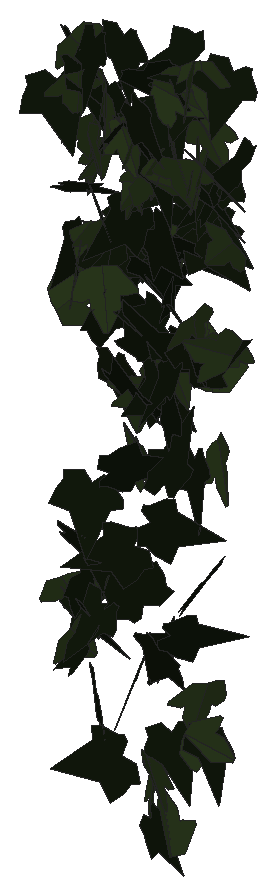
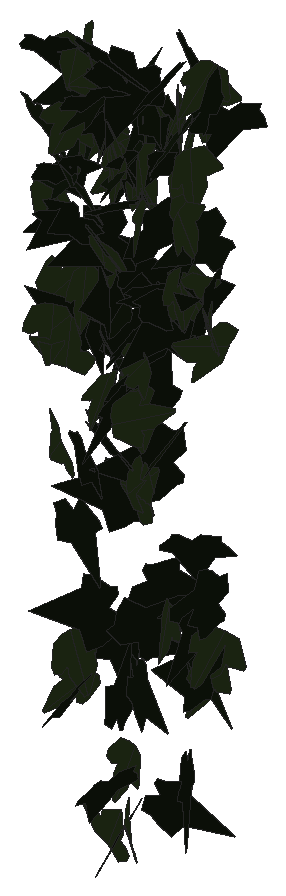
# SketchUp Ruby script. Lengths in inches.
U = 1.inch
M = Sketchup.active_model
def pt(a) = Geom::Point3d.new(a.map { |v| v * U })
def face(e, loops, mat)
  f = e.add_face(loops[0].map { |a| pt(a) })
  loops[1..].each { |l| e.add_face(l.map { |a| pt(a) }).erase! }
  f.material = f.back_material = mat if mat
  f
end
# faces: each face lists its corners as indices into pts; further lists are holes
def faces(e, pts, list, mat = nil) = list.each { |f| face(e, (f[0].is_a?(Array) ? f : [f]).map { |l| l.map { |i| pts[i] } }, mat) }
# xy, xz, yz: faces in a plane at the given z, y or x. An outline is a flat list of corners, or four numbers for a rectangle; further outlines are holes
def ring(l) = l.size == 4 ? [[l[0], l[1]], [l[2], l[1]], [l[2], l[3]], [l[0], l[3]]] : l.each_slice(2).to_a
def flat(e, list, mat, &to3) = list.each { |f| face(e, (f[0].is_a?(Array) ? f : [f]).map { |l| ring(l).map { |u, v| to3.(u, v) } }, mat) }
def xy(e, z, list, mat = nil) = flat(e, list, mat) { |x, y| [x, y, z] }
def xz(e, y, list, mat = nil) = flat(e, list, mat) { |x, z| [x, y, z] }
def yz(e, x, list, mat = nil) = flat(e, list, mat) { |y, z| [x, y, z] }
def lines(e, pts, list) = list.each { |a, b| e.add_line(pt(pts[a]), pt(pts[b])) }
# prism: a flat outline (further loops are holes) pulled along v
def prism(e, loops, v, mat = nil)
  f = face(e, loops, mat); d = Geom::Vector3d.new(v.map { |x| x * U })
  f.pushpull(f.normal.samedirection?(d) ? d.length : -d.length)
end
def box(e, o, s, mat = nil) = prism(e, [[o, [o[0] + s[0], o[1], o[2]], [o[0] + s[0], o[1] + s[1], o[2]], [o[0], o[1] + s[1], o[2]]]], [0, 0, s[2]], mat)
def at(x, y, z, deg = 0) = Geom::Transformation.translation(pt([x, y, z])) * Geom::Transformation.rotation(ORIGIN, Z_AXIS, deg.degrees)
def axes(o, x, y, z) = Geom::Transformation.new([*x, 0, *y, 0, *z, 0, *pt(o).to_a, 1])
def part(name) = M.definitions.add(name)
# library, detail: a bought-in or finely detailed component or shape, given as its bounding box
def library(name, o, s) = part(name).tap { |d| box(d.entities, o, s) }
def detail(e, o, s) = box(e.add_group.entities, o, s)
def put(e, d, t, mat = nil) = e.add_instance(d, t).tap { |i| i.material = mat if mat }
def group(e, t, mat = nil) = e.add_group.tap { |g| g.transformation = t; g.material = mat if mat }.entities
root = M.entities
M.materials.add("efeu1").color = [18, 25, 13]
M.materials.add("efeu2").color = [43, 57, 29]
c1 = part("ivyleaf_10")
p = [[0,0.5,-0.03],[-0.0625,2.02,-0.43],[-0.19,2.01,-0.46],[-0.54,1.05,-0.29],[-0.52,0.625,-0.18],[-0.83,0.76,-0.28],
  [-1.16,0.64,-0.33],[-1.15,0.33,-0.24],[-0.77,-0.39,0.02],[-0.3,-0.51,0.16],[0.04,-0.48,0.23],[-0.02,2.01,-0.4375],
  [-0.06,2.01,-0.43],[0.04,-0.49,0.23],[0.67,-0.49,0.14],[1.38,0.36,-0.2],[1.375,0.51,-0.24],[0.81,0.65,-0.19],
  [0.62,0.59,-0.15],[0.6,1.09,-0.28],[0.5,1.23,-0.31]]
faces(c1.entities,p,[[0,1,2,3,4,5,6,7,8,9,10],[11,12,0,13,14,15,16,17,18,19,20]],"efeu2")
c2 = part("ivyleaf_9")
p = [[1.54,2.16,1.25],[1.36,2.04,1.19],[-0.21,0.99,0.68],[-0.71,1.11,0.82],[-0.85,0.86,0.67],[-0.8,0.17,0.21],
  [-0.9,-0.01,0.1],[-0.67,-0.16,-0.02],[-0.08,-0.08,-0.05],[-0.03,-0.6,-0.4],[0.65,-0.88,-0.66],[0.83,-0.6,-0.49],
  [1.29,-0.42,-0.43],[1.8125,-0.07,-0.26],[1.21,0.44,0.15]]
faces(c2.entities,p,[[0,1,2,3,4,5,6,7,8,9,10,11,12,13,14]],"efeu1")
put(root,c1,axes([569.7,129.61,232.22],[0.70145,-0.65634,0.53358],[0.41076,-0.34165,-0.96025],[0.73944,0.81242,0.02725]))
put(root,c1,axes([569.9,128.73,216.94],[-0.81797,-0.47877,-0.41518],[0.36479,0.1986,-0.94771],[0.51819,-0.89555,0.01179]))
put(root,c2,axes([569.78,128.19,241.03],[-0.27032,-0.84002,-0.601],[0.16207,0.57905,-0.88223],[1.02008,-0.3146,-0.0191]))
put(root,c2,axes([569.79,129.69,232.91],[0.1482,-0.311,-1.0442],[0.74854,-0.73667,0.32565],[-0.79168,-0.75474,0.11243]))
put(root,c2,axes([570.59,129.82,211.49],[0.42167,-0.05463,-1.11509],[-1.09323,0.22152,-0.42426],[0.2264,1.1714,0.02823]))
put(root,c1,axes([570.12,130.67,236.97],[0.1507,-0.92178,0.36124],[0.17028,-0.33582,-0.92796],[0.97528,0.20107,0.1062]))
put(root,c2,axes([569.73,129.04,235.75],[0.88828,0.23998,0.34562],[0.22936,0.4007,-0.86771],[-0.35276,0.86483,0.30613]))
put(root,c1,axes([569.89,128.67,230.47],[0.39278,0.28681,-1.10408],[0.51317,0.99844,0.44193],[1.01877,-0.61351,0.20306]))
put(root,c2,axes([569.57,129.75,241.78],[0.26671,-0.44193,0.88519],[0.48053,-0.74354,-0.51599],[0.86485,0.54941,0.01372]))
put(root,c1,axes([570.59,129.89,233.33],[-0.45692,-0.70836,0.4892],[-0.1154,-0.49844,-0.82953],[0.8531,-0.44682,0.14981]))
put(root,c1,axes([570.21,128.92,242.9],[-0.37135,-0.69007,-0.62037],[0.40349,0.48164,-0.77729],[0.83562,-0.53924,0.09963]))
put(root,c2,axes([569.68,129.15,218.99],[0.86105,-0.30925,0.40015],[0.38726,-0.10497,-0.91443],[0.32525,0.94367,0.02942]))
put(root,c1,axes([570.64,129.47,239],[-0.22391,-1.02151,-0.09899],[0.01457,0.09814,-1.04574],[1.02619,-0.22428,-0.00675]))
put(root,c1,axes([570.75,129.94,233.77],[-0.21913,-0.97227,-0.07492],[0.02507,0.07114,-0.99662],[0.97483,-0.22038,0.00879]))
put(root,c2,axes([570.72,128.7,217.71],[0.14322,-0.1899,-1.0038],[-0.57223,0.82477,-0.23768],[0.8463,0.58981,0.00917]))
put(root,c1,axes([570.92,128.19,241.61],[-0.50756,-0.88923,-0.05619],[0.03307,0.04582,-1.02387],[0.89039,-0.5086,0.006]))
put(root,c1,axes([570.78,128.12,215.17],[-0.20716,-0.80324,-0.61711],[0.23526,0.5745,-0.82676],[0.98522,-0.30608,0.06766]))
put(root,c2,axes([570.33,129.01,241.64],[0.54254,-0.88522,-0.02887],[-0.01396,0.0253,-1.03825],[0.88558,0.54272,0.00132]))
put(root,c2,axes([570.66,129.38,221.59],[-0.57973,-0.74969,-0.43056],[0.30313,0.30922,-0.94657],[0.80965,-0.65257,0.0461]))
put(root,c2,axes([570.08,129.18,215.6],[0.78487,-0.54343,0.64876],[0.53371,-0.36884,-0.95464],[0.65678,0.94914,0.00047]))
put(root,c1,axes([570.99,130.01,237.6],[-0.22351,0.2623,-0.98467],[-0.12785,-1.00733,-0.23932],[-1.01096,0.0694,0.24796]))
put(root,c2,axes([571.57,127.96,215.02],[-0.69099,0.71685,0.04568],[-0.03258,0.03204,-0.99566],[-0.71757,-0.69175,0.00122]))
put(root,c2,axes([570.57,131.12,226.69],[0.39898,-0.90696,0.08901],[0.02824,-0.08481,-0.9908],[0.91087,0.3999,-0.00827]))
put(root,c2,axes([570.7,129.96,234.38],[0.00644,-0.28757,0.95768],[0.29716,-0.91388,-0.27642],[0.95474,0.28638,0.07957]))
put(root,c2,axes([571.5,128.86,216.42],[-0.8605,-0.3948,-0.10499],[0.09426,0.04632,-0.94674],[0.39749,-0.86564,-0.00277]))
put(root,c2,axes([570.86,130.35,240.21],[0.30381,-0.94323,0.32201],[0.09905,-0.3064,-0.99095],[0.99174,0.31955,0.00033]))
put(root,c2,axes([572.23,129.27,209.27],[-0.16556,-0.18541,-1.08955],[-0.78643,-0.75432,0.24786],[-0.77655,0.80345,-0.01873]))
put(root,c1,axes([571.625,129.67,218.02],[0.13472,-0.64866,-0.7827],[-0.11772,0.77428,-0.66194],[1.00971,0.17682,0.02726]))
put(root,c1,axes([571.63,128.95,241.01],[0.47628,-0.66587,-0.57347],[-0.17406,0.56788,-0.80394],[0.86137,0.48293,0.15464]))
put(root,c2,axes([572.26,130.57,232.38],[-0.18477,0.08846,0.99512],[-0.93446,0.34265,-0.20396],[-0.35337,-0.95236,0.01905]))
put(root,c2,axes([571.53,129.76,232.95],[-0.78249,-0.51324,-0.4636],[0.41144,0.21725,-0.93496],[0.55593,-0.88318,0.03943]))
put(root,c2,axes([571.49,128.5625,243.46],[-0.71582,0.02079,-0.74056],[0.73964,-0.03885,-0.71602],[-0.04238,-1.02923,0.01207]))
put(root,c1,axes([571.88,127.95,239.05],[-0.55913,0.7616,0.28988],[-0.20836,0.20626,-0.94379],[-0.78782,-0.59508,0.04387]))
put(root,c2,axes([571.43,130.57,242.72],[0.18374,-0.99056,0.1031],[0.01003,-0.103,-1.00742],[0.99586,0.1838,-0.00887]))
put(root,c2,axes([572.39,130.92,232.9],[-0.7279,-0.32585,0.53966],[-0.36753,-0.45038,-0.76767],[0.51219,-0.78627,0.21608]))
put(root,c2,axes([572.11,131.05,234.21],[-0.62378,-0.71816,0.13],[-0.09271,-0.09165,-0.95119],[0.72391,-0.63056,-0.0098]))
put(root,c2,axes([572.55,129.69,219.22],[-0.191,-0.22183,-0.99104],[-0.26268,-0.96331,0.26625],[-0.98101,0.30113,0.12166]))
put(root,c1,axes([571.93,131.07,239.15],[0.29654,-0.85145,0.44654],[0.44464,-0.29287,-0.85371],[0.85245,0.44895,0.28996]))
put(root,c1,axes([571.98,128.86,240.53],[-0.16508,0.58169,-0.82619],[0.27248,-0.7805,-0.60397],[-0.97299,-0.31726,-0.02897]))
put(root,c2,axes([572.25,128.43,231.17],[-0.04017,0.06913,-1.16094],[-0.32256,1.1154,0.07758],[1.11737,0.32448,-0.01934]))
put(root,c2,axes([572.88,129.93,216.58],[0.24328,0.06255,1.08971],[-1.07655,-0.17041,0.25013],[0.18005,-1.10346,0.02314]))
put(root,c1,axes([572.17,128.19,232.49],[0.97439,0.48063,0.2078],[0.18553,0.09361,-1.08648],[-0.48966,0.9919,0.00185]))
put(root,c1,axes([572.69,130.03,236.48],[-0.41785,0.74822,0.45618],[-0.30859,0.34737,-0.85243],[-0.82019,-0.51189,0.08832]))
put(root,c2,axes([572.34,130.36,238.98],[-0.30253,-0.80343,-0.59031],[0.27605,0.52526,-0.85637],[0.958,-0.40507,0.06036]))
put(root,c1,axes([573.25,130.48,226.74],[-0.09785,-0.05734,-0.98275],[-0.83384,-0.52011,0.11337],[-0.52326,0.83955,0.00311]))
put(root,c1,axes([573.25,129.76,223.28],[-0.60691,0.33695,-0.68674],[-0.60044,0.33329,0.69418],[0.47394,0.85374,0.00005]))
put(root,c2,axes([572.71,129.77,235.31],[0.00185,-0.20098,-1.11062],[0.43957,-1.0228,0.18582],[-1.03954,-0.43285,0.0766]))
put(root,c2,axes([573.11,128.5,240.18],[-0.35813,0.92104,-0.16784],[0.05606,-0.15828,-0.9882],[-0.93453,-0.36245,0.00503]))
put(root,c1,axes([572.73,130.2,229.37],[-0.69174,0.30846,-0.60263],[0.5023,-0.34379,-0.75254],[-0.45388,-0.85057,0.08563]))
put(root,c1,axes([572.4,130.15,223.17],[0.01626,-0.11636,1.02492],[1.01253,-0.19391,-0.03808],[0.19694,1.00654,0.11115]))
put(root,c2,axes([572.67,131.14,238.75],[0.47533,-0.87456,0.13595],[0.09502,-0.103,-0.99481],[0.87995,0.48354,0.03398]))
put(root,c1,axes([573.35,128.94,239.49],[0.40666,-0.89437,-0.35702],[-0.10912,0.34226,-0.98168],[0.95679,0.41916,0.03978]))
put(root,c2,axes([573.13,130.56,238.34],[-0.73137,-0.05491,-0.66628],[0.66854,-0.06017,-0.72889],[-0.00007,-0.98753,0.08146]))
put(root,c1,axes([573.47,129.51,227.01],[-0.40901,-0.94121,0.11609],[-0.02788,-0.11444,-1.02605],[0.94794,-0.40947,0.01991]))
put(root,c2,axes([573.36,129.65,214.42],[-0.69951,0.41779,-0.85188],[0.70646,-0.47716,-0.81412],[-0.63337,-0.99365,0.03277]))
put(root,c2,axes([573.19,129.04,226.78],[1.00738,-0.51988,0.29536],[-0.25351,0.15271,1.13347],[-0.54152,-1.03862,0.01882]))
put(root,c1,axes([573.34,129.54,237.5],[0.08209,-0.90941,0.49107],[0.14866,-0.4771,-0.90839],[1.02277,0.14234,0.09262]))
put(root,c1,axes([573.54,130.58,238.74],[-0.83868,0.49111,0.21229],[-0.20586,0.06814,-0.97089],[-0.49384,-0.86245,0.04418]))
put(root,c2,axes([573.23,130.96,213.47],[0.08045,0.38579,0.9606],[-0.2994,-0.91364,0.39201],[0.99093,-0.30737,0.04045]))
put(root,c2,axes([573.13,128.64,239.84],[0.96582,-0.05279,-0.27389],[-0.27354,0.01388,-0.96726],[0.05458,1.00381,-0.00103]))
put(root,c1,axes([573.17,129.5,237.2],[-0.23553,-0.22752,0.99468],[0.48944,-0.92092,-0.09475],[0.89532,0.44358,0.31346]))
put(root,c1,axes([572.99,130.55,208.08],[0.49465,-0.46315,0.75785],[0.59801,-0.4677,-0.67614],[0.65668,0.77478,0.04488]))
put(root,c2,axes([573.4,129.6,242.22],[0.72248,0.84775,-0.11153],[-0.0758,-0.08193,-1.11384],[-0.85169,0.72643,0.00452]))
put(root,c1,axes([572.92,128.51,239.74],[0.84175,0.0159,0.54691],[0.54134,0.12165,-0.8367],[-0.07952,0.99642,0.09342]))
put(root,c2,axes([573.66,131.29,236.63],[-0.71664,-0.52105,0.38349],[-0.07986,-0.49666,-0.82406],[0.64201,-0.6434,0.32556]))
put(root,c2,axes([573.58,130.46,229.74],[0.25344,-0.93383,-0.33429],[0.1158,-0.31481,0.96721],[-0.98508,-0.27727,0.0277]))
put(root,c2,axes([573.03,127.89,223.76],[0.56915,0.28094,0.92733],[0.8215,0.43039,-0.63459],[-0.51382,0.99932,0.0126]))
put(root,c2,axes([573.89,129.3125,229.1875],[0.69706,-0.06657,0.72988],[-0.71726,0.1451,0.69824],[-0.15066,-0.99878,0.05279]))
put(root,c1,axes([573.65,130.92,240.18],[0.73479,-0.64544,0.17662],[0.13276,-0.11649,-0.97801],[0.65587,0.74668,0.00009]))
put(root,c2,axes([573.71,129.92,227.48],[0.4635,-0.57586,-0.8525],[-0.44206,0.73282,-0.73536],[0.92895,0.63605,0.07542]))
put(root,c2,axes([573.26,130.23,231.89],[0.72209,-0.63325,0.29637],[0.22417,-0.19388,-0.96043],[0.66226,0.75608,0.00195]))
put(root,c2,axes([574.11,130.22,227.17],[-0.2662,-0.55305,0.78255],[-0.38648,-0.68124,-0.61292],[0.87686,-0.46816,-0.03257]))
put(root,c2,axes([574.01,129.13,233.37],[0.86505,0.46181,-0.34816],[-0.3032,-0.1713,-0.98057],[-0.4925,0.91661,-0.00785]))
put(root,c2,axes([574.61,130.68,234.78],[-0.85629,0.46454,0.01801],[-0.01323,0.01337,-0.97417],[-0.46471,-0.85637,-0.00545]))
put(root,c2,axes([573.76,130.89,210.11],[0.10816,-0.95763,-0.34904],[-0.00827,0.35016,-0.96327],[1.01922,0.10446,0.02922]))
put(root,c1,axes([574.2,129.85,238.41],[0.29948,-0.94668,0.22063],[0.06489,-0.21088,-0.99292],[0.96988,0.30642,-0.00169]))
put(root,c2,axes([573.72,129.96,237.73],[0.34986,-0.92528,0.22306],[0.07253,-0.21105,-0.9892],[0.94902,0.35724,-0.00663]))
put(root,c2,axes([573.96,130.16,240.43],[-0.01354,-0.98001,-0.37608],[-0.00905,0.37621,-0.98001],[1.04965,-0.00939,-0.0133]))
put(root,c2,axes([574.43,129.75,231.59],[0.08668,0.29612,1.08571],[0.23877,1.0593,-0.30797],[-1.09975,0.25333,0.01871]))
put(root,c2,axes([575.09,130.5,242.97],[-0.88933,0.28049,0.42264],[-0.42587,0.05053,-0.92966],[-0.27555,-0.98335,0.07278]))
put(root,c2,axes([574.01,128.07,241.25],[0.71317,-0.67532,-0.39492],[-0.28945,0.26869,-0.98217],[0.7268,0.76966,-0.00364]))
put(root,c1,axes([574.33,130.37,228],[-0.13303,0.94291,0.28828],[-0.07672,0.28011,-0.95159],[-0.983,-0.14946,0.03526]))
put(root,c1,axes([574.12,128.84,237.75],[-0.40307,-0.46862,-0.85608],[0.53543,0.66821,-0.61787],[0.81597,-0.66996,-0.01745]))
put(root,c1,axes([574.25,130.52,234.19],[0.94176,-0.18503,0.16172],[0.15628,-0.04339,-0.95969],[0.18965,0.95456,-0.01228]))
put(root,c2,axes([574.49,131.33,241.46],[-0.57099,-0.82078,-0.06248],[0.10045,0.006,-0.99674],[0.817,-0.57437,0.07888]))
put(root,c2,axes([575.01,128.46,215.64],[0.53909,0.2843,-0.86239],[-0.83776,-0.23116,-0.5999],[-0.35028,0.9904,0.10753]))
put(root,c1,axes([574.62,128.54,210],[-0.9403,0.45231,-0.11184],[0.097,-0.05635,-1.0434],[-0.45573,-0.94525,0.00868]))
put(root,c2,axes([574.47,128.72,207.21],[0.60644,-0.58438,-0.50934],[-0.35078,0.36982,-0.84195],[0.69129,0.70031,0.01959]))
put(root,c2,axes([574.34,130.72,241.34],[0.81136,-0.57448,-0.09652],[-0.06955,0.06878,-0.99402],[0.57837,0.81418,0.01587]))
put(root,c1,axes([575.15,129.125,206.32],[1.00963,-0.13683,0.58896],[-0.58218,0.08956,1.01882],[-0.16327,-1.16542,0.00914]))
put(root,c1,axes([574.05,129.96,241.34],[0.17193,0.10037,1.09442],[1.02617,0.38191,-0.19624],[-0.39345,1.03993,-0.03357]))
put(root,c1,axes([574.89,129.58,239.23],[-0.54877,0.79665,-0.17631],[0.08082,-0.15836,-0.9671],[-0.81192,-0.55422,0.0229]))
put(root,c2,axes([575.22,128.72,227.37],[0.42709,-0.24428,-0.92315],[-0.79574,0.46801,-0.49199],[0.5279,0.90309,0.00525]))
put(root,c2,axes([575.34,129.04,229.1],[-0.90727,0.33822,-0.45101],[0.41706,-0.17226,-0.96816],[-0.37929,-0.99843,0.01426]))
put(root,c2,axes([574.44,129.62,234.31],[0.96631,0.03973,0.39257],[0.39148,0.03333,-0.967],[-0.04934,1.04248,0.01596]))
put(root,c2,axes([575.19,128.72,223.72],[-0.84435,0.68941,0.28292],[0.21616,-0.18259,1.09004],[0.71316,0.87157,0.00457]))
put(root,c2,axes([575.43,127.72,236.12],[0.50504,-0.45378,-0.89868],[-0.70063,0.56358,-0.67831],[0.72295,0.86317,-0.02957]))
put(root,c2,axes([576.16,128.98,230.33],[0.42661,0.16061,-0.87581],[-0.86468,-0.15706,-0.44999],[-0.21251,0.96144,0.07279]))
put(root,c2,axes([574.9375,128.18,221.8125],[0.48791,0.12942,-0.95774],[0.5732,0.82505,0.4035],[0.77812,-0.68893,0.3033]))
put(root,c1,axes([575.58,129.86,242.8],[0.56168,-0.66441,0.50846],[0.37999,-0.34301,-0.86799],[0.74537,0.67554,0.05935]))
put(root,c1,axes([575.76,130.76,239.8],[-0.89115,-0.15315,-0.37504],[0.39299,-0.10685,-0.89016],[0.09833,-0.96092,0.15876]))
put(root,c2,axes([575.63,130.04,224.17],[-0.50078,-0.05464,-0.90576],[0.90507,0.04422,-0.50306],[0.06517,-1.03404,0.02635]))
put(root,c1,axes([576.18,129.44,239.01],[0.33798,-0.75033,-0.66937],[-0.13101,0.66729,-0.81415],[0.99694,0.34207,0.11993]))
put(root,c2,axes([576.52,130.23,237.24],[-0.80491,0.56318,-0.06811],[0.06643,-0.02384,-0.98219],[-0.56338,-0.80743,-0.01851]))
put(root,c1,axes([576.15,128.57,239.0625],[-1.02256,-0.28227,-0.10508],[0.10145,0.02737,-1.06081],[0.28359,-1.02758,0.00061]))
put(root,c2,axes([576.11,131.09,237.64],[-0.58791,-0.78595,-0.12915],[0.07839,0.10264,-0.98151],[0.79263,-0.59311,0.00128]))
put(root,c1,axes([575.83,130.2,242.73],[0.95705,0.15262,0.27487],[0.23454,0.23996,-0.94984],[-0.20938,0.96639,0.19244]))
put(root,c1,axes([576.27,129.1875,231.49],[-0.15479,-0.98608,-0.33996],[0.06561,0.3338,-0.99808],[1.04097,-0.16767,0.01236]))
put(root,c2,axes([575.54,130.68,235.3125],[0.1315,-0.39991,-0.89106],[0.64016,0.71433,-0.22612],[0.73763,-0.54864,0.35509]))
put(root,c2,axes([575.64,128.68,216.51],[0.23825,0.54284,-0.87349],[0.36877,0.7919,0.59272],[0.96004,-0.43891,-0.0109]))
put(root,c1,axes([576.39,130.31,228.41],[1.0876,0.29269,0.18353],[-0.17757,-0.04641,1.12629],[0.29634,-1.102,0.00131]))
put(root,c1,axes([576.45,129.54,238.92],[0.68183,-0.83053,0.233],[0.14428,-0.18302,-1.07455],[0.85045,0.69691,-0.00451]))
put(root,c2,axes([575.98,130.51,234.91],[-0.00989,-0.55376,-0.81589],[0.49182,0.70442,-0.48407],[0.85466,-0.41177,0.26912]))
put(root,c2,axes([575.99,130.26,237.16],[0.63751,-0.69179,0.2791],[0.2946,-0.10382,-0.93022],[0.68533,0.68814,0.14024]))
put(root,c1,axes([577.08,130.41,230.11],[-0.94714,-0.23174,0.09144],[-0.08663,-0.03069,-0.97504],[0.23359,-0.95105,0.00919]))
put(root,c2,axes([576.2,129.2,229.23],[-0.0553,0.02805,1.04957],[1.04022,-0.14123,0.05859],[0.14255,1.04149,-0.02032]))
put(root,c1,axes([576.35,130.65,224.61],[0.67139,-0.27247,0.87737],[0.81848,-0.31617,-0.72451],[0.41727,1.05858,0.00944]))
put(root,c1,axes([577.21,128.74,214.35],[-0.38728,-1.02299,0.20415],[-0.06385,-0.19411,-1.09381],[1.0412,-0.39241,0.00886]))
put(root,c2,axes([577.01,130.78,242.875],[-0.72946,-0.60821,-0.28835],[0.27707,0.11619,-0.946],[0.61344,-0.77574,0.08439]))
put(root,c2,axes([577.58,128.23,219.96],[-0.4504,0.94914,-0.14608],[0.06352,-0.13154,-1.05058],[-0.95821,-0.45486,-0.00099]))
put(root,c1,axes([577.85,129.59,235.46],[-0.68629,-0.1043,0.71245],[-0.70563,-0.09855,-0.69414],[0.14337,-0.98431,-0.00599]))
put(root,c1,axes([577.85,129.23,230.48],[-0.3229,-0.39598,-0.93235],[-0.56837,-0.73918,0.51078],[-0.83846,0.65357,0.01281]))
put(root,c2,axes([578.13,129.94,239.02],[-0.60007,0.72192,0.3168],[-0.22296,0.22648,-0.93841],[-0.75619,-0.63965,0.02529]))
put(root,c2,axes([577.15,129.13,212.08],[0.22145,-1.02238,0.08636],[0.0275,-0.0824,-1.04605],[1.02566,0.22295,0.0094]))
put(root,c1,axes([577.3,128.03,212.39],[0.19151,0.53619,0.82078],[0.27557,0.77314,-0.56937],[-0.94088,0.33558,0.00031]))
put(root,c2,axes([577.17,128.26,239.87],[0.84558,-0.47929,0.22331],[0.22883,-0.048,-0.9695],[0.47668,0.87325,0.06928]))
